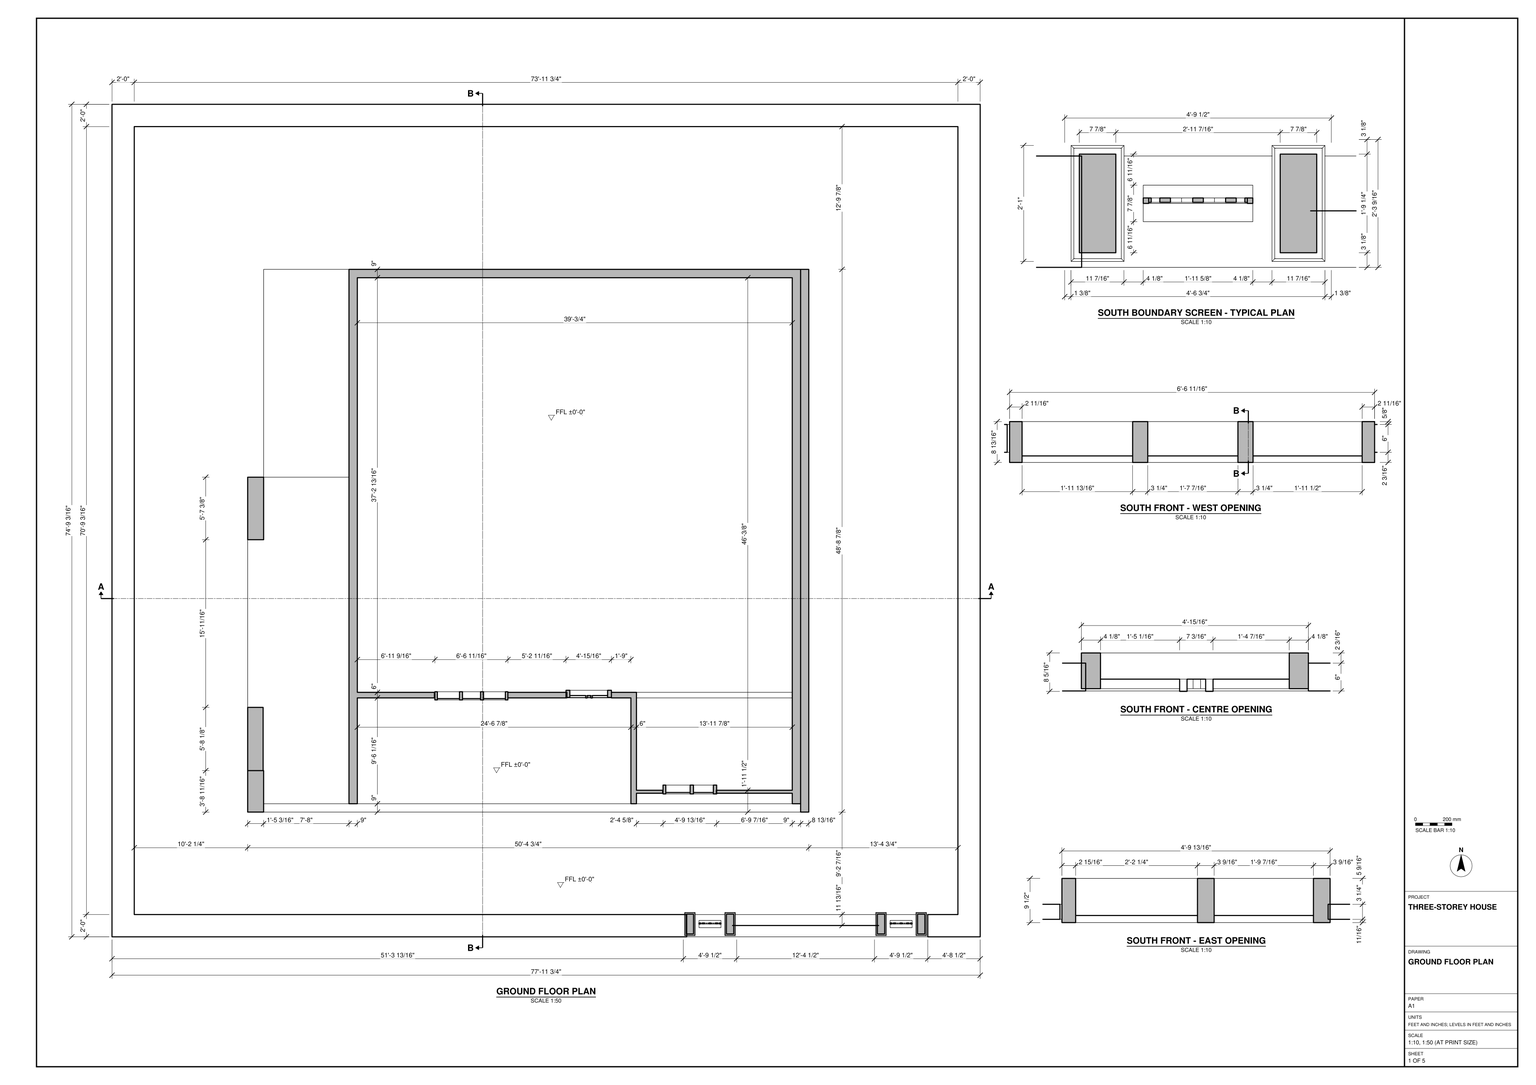
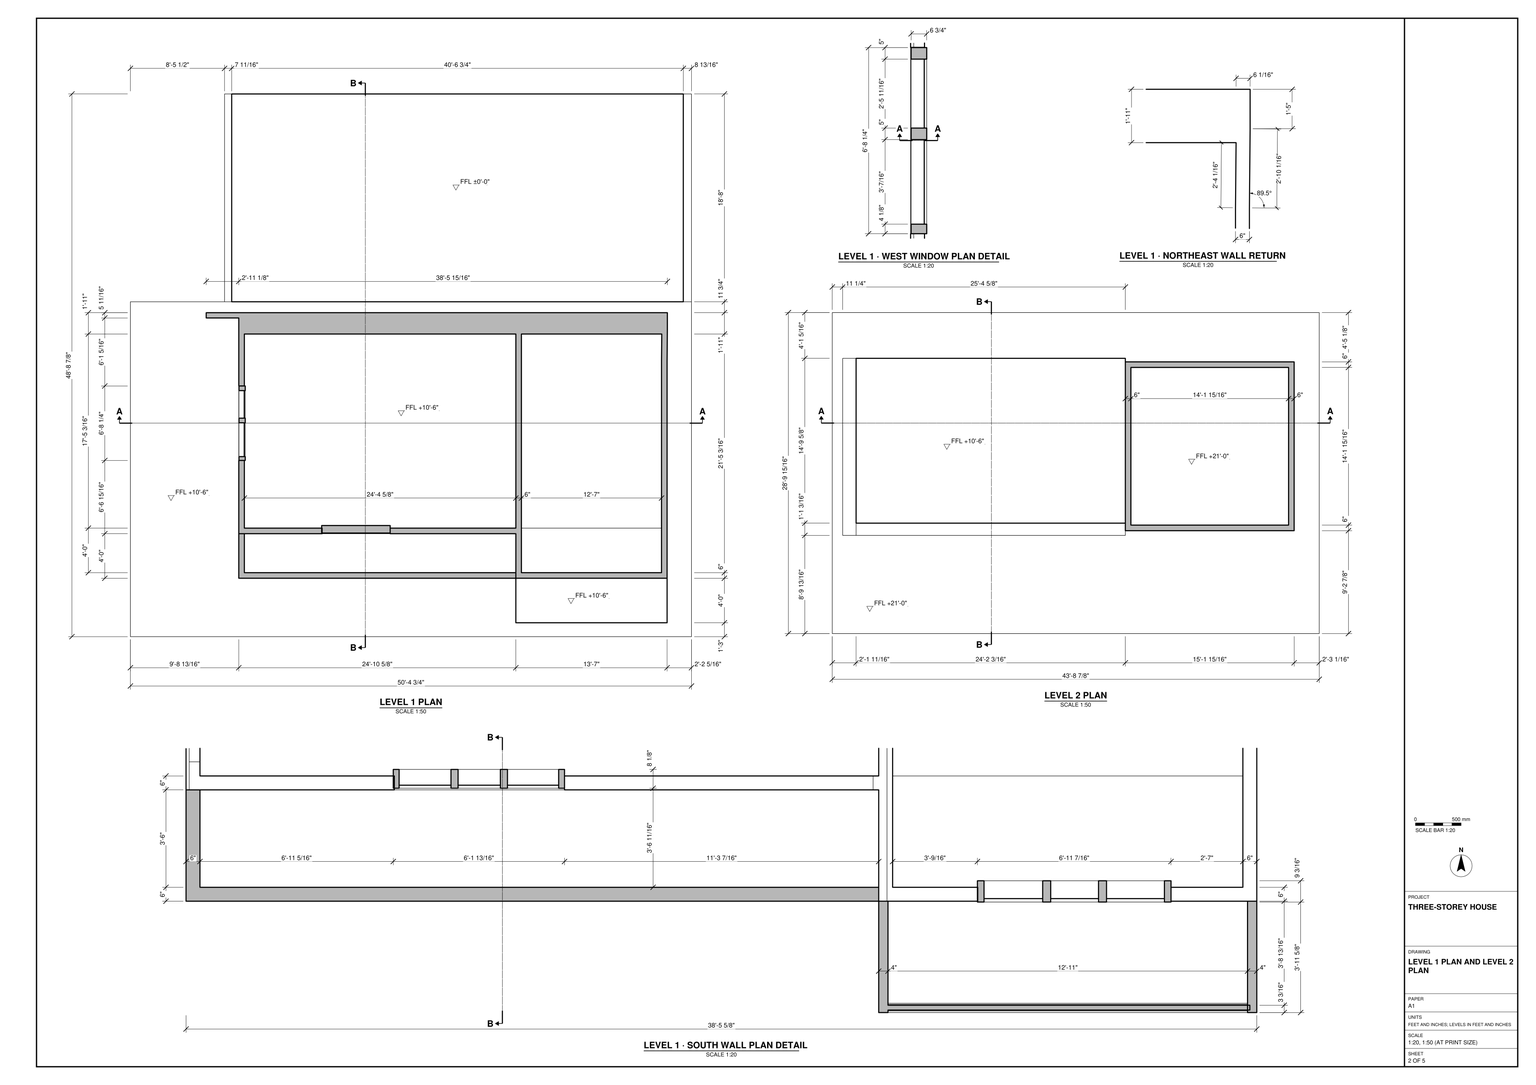
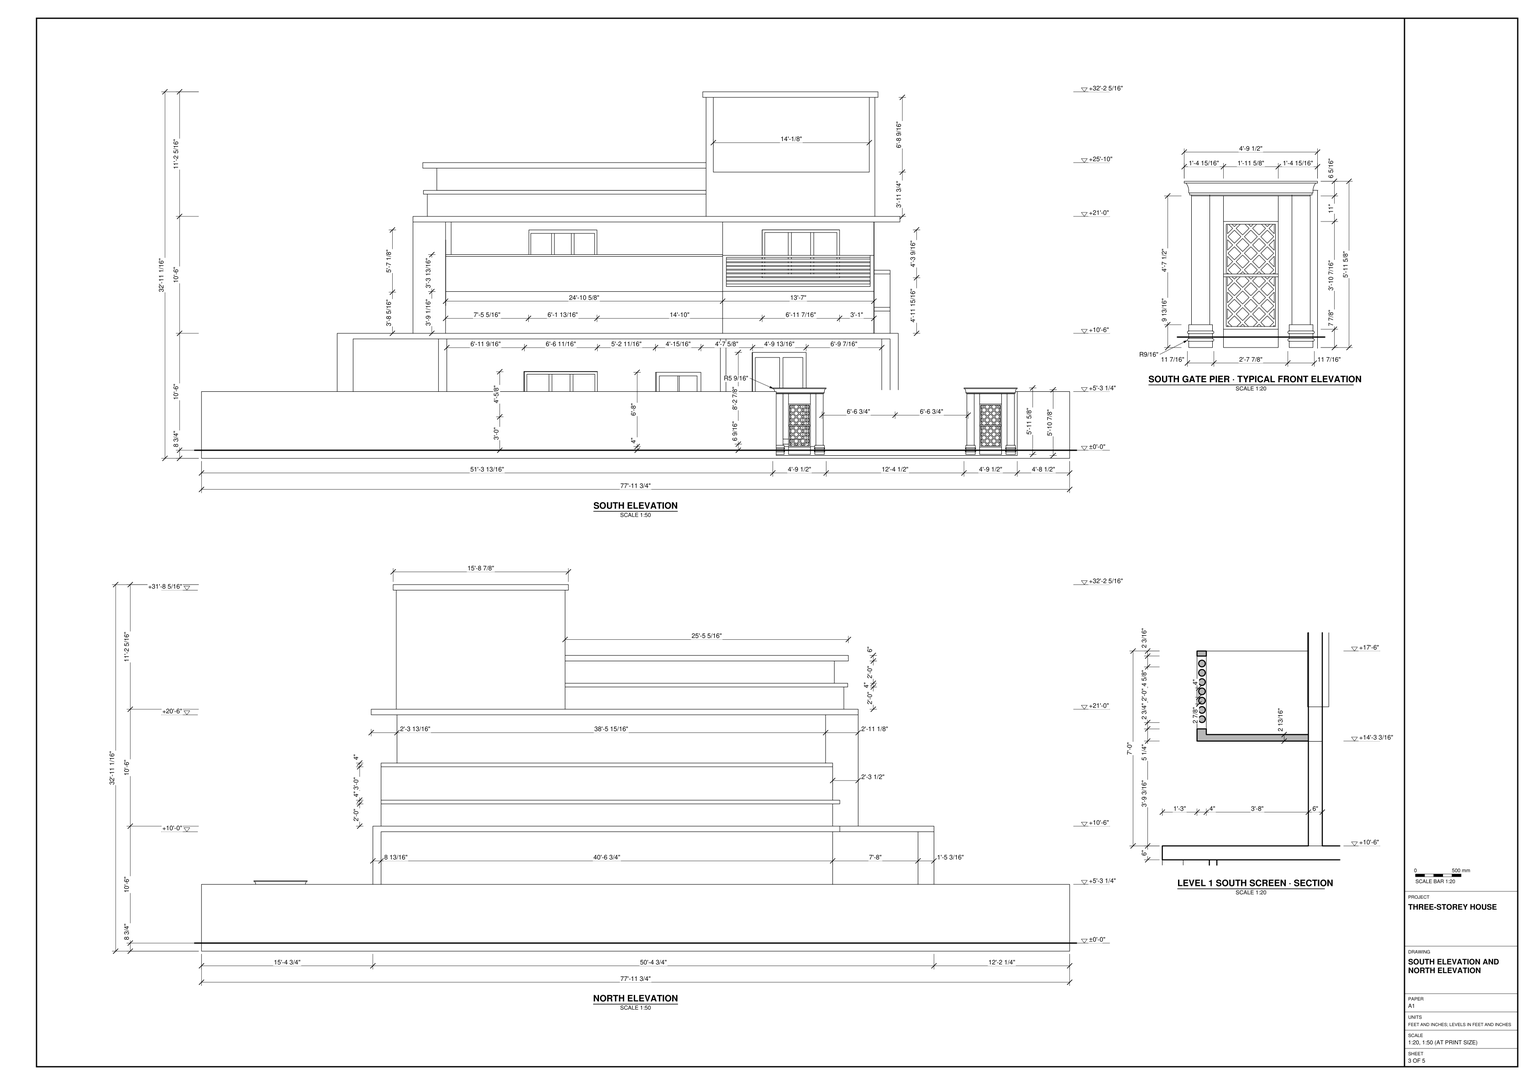
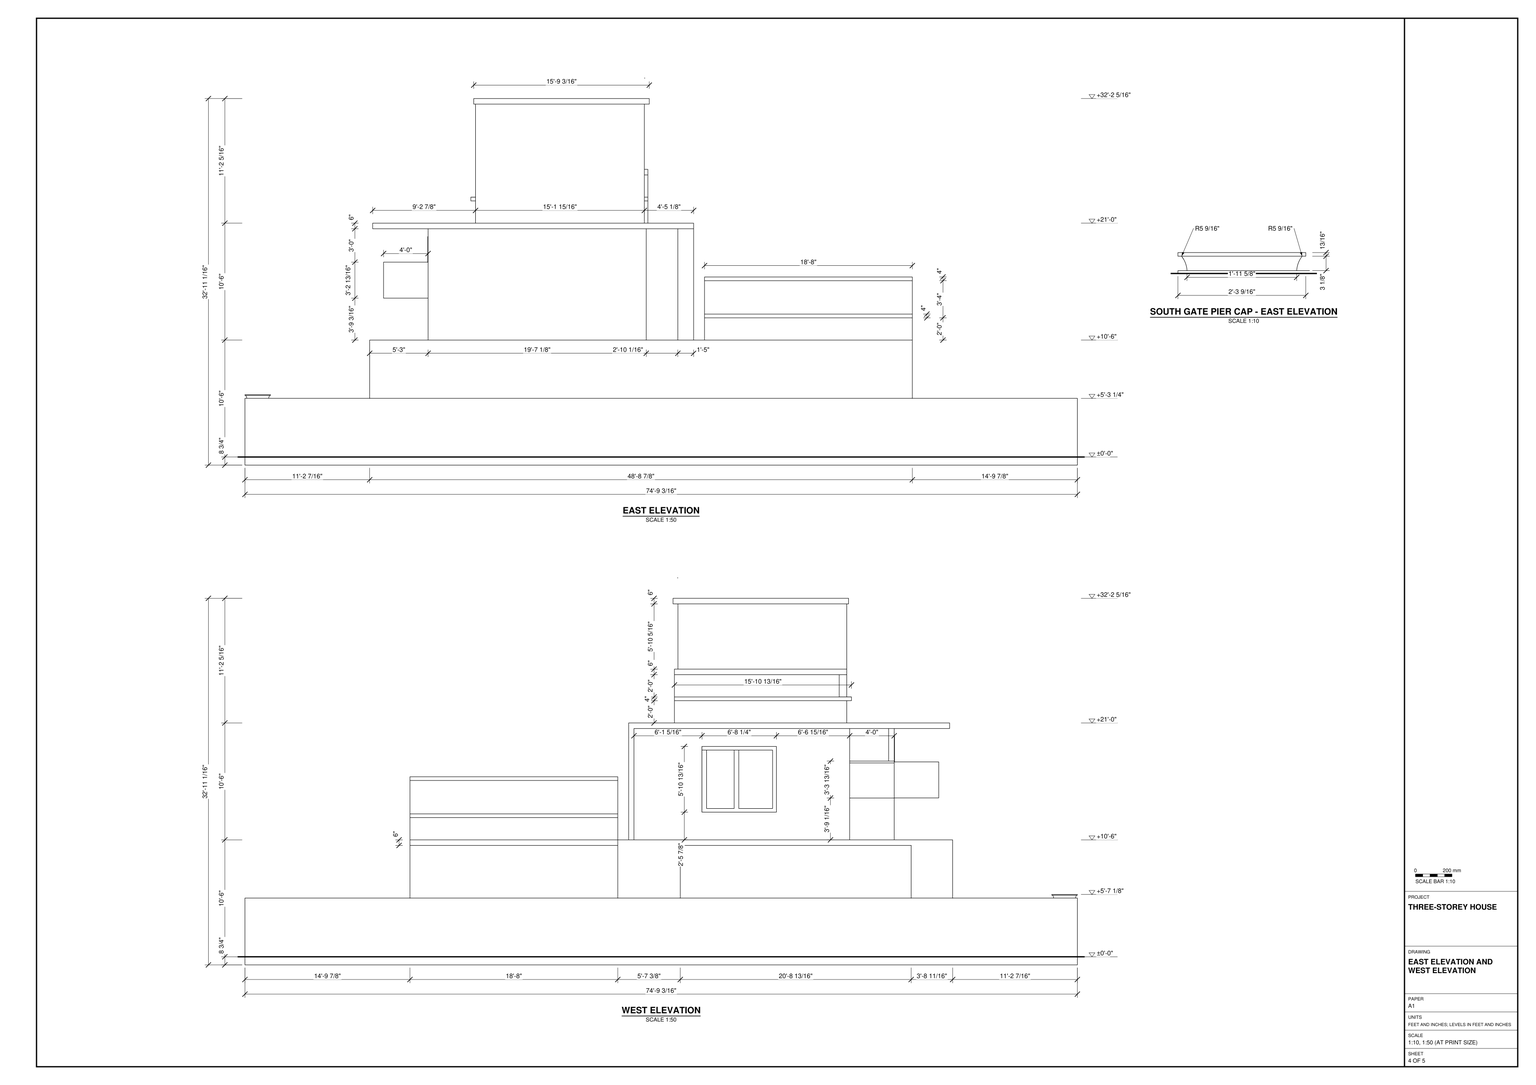
Build the house and its site in SketchUp from task_files/diagram_01.pdf. Work in feet and inches. The full model, including the site boundary, measures 77'-11 3/4" east to west, 74'-9 3/16" north to south and 32'-11 1/16" in height. Set the finished floor levels to ±0'-0", +10'-6" and +21'-0".

Use the ground floor plan to position the house within the boundary walls. Model the stepped south frontage, its framed openings and the slab projection with supports on the west side. Along the south boundary, place the two lattice screens between their capped piers as shown in the plan and elevation. Follow the drawn wall thicknesses, including the 9" ground floor exterior walls and the 6" walls where indicated, rather than using one thickness throughout.

Use the upper floor plans to locate the slabs, wall returns and setbacks. On the first upper floor, distinguish the solid balcony front from the projecting section with horizontal screening. On the top floor, place the taller enclosure to the east of the lower roof and carry the projecting flat roof edges around the volumes as drawn.

Keep walls, slabs, roofs and any furniture or joinery pieces in separate groups or components, and use components for repeated parts. Any decor or loose items shown may be represented by suitable library components. Save one SketchUp model as output_files/three_storey_house_and_its_walled_site.skp.

# SketchUp Ruby script. Lengths in inches.
U = 1.inch
M = Sketchup.active_model
def pt(a) = Geom::Point3d.new(a.map { |v| v * U })
def face(e, loops, mat)
  f = e.add_face(loops[0].map { |a| pt(a) })
  loops[1..].each { |l| e.add_face(l.map { |a| pt(a) }).erase! }
  f.material = f.back_material = mat if mat
  f
end
# faces: each face lists its corners as indices into pts; further lists are holes
def faces(e, pts, list, mat = nil) = list.each { |f| face(e, (f[0].is_a?(Array) ? f : [f]).map { |l| l.map { |i| pts[i] } }, mat) }
# xy, xz, yz: faces in a plane at the given z, y or x. An outline is a flat list of corners, or four numbers for a rectangle; further outlines are holes
def ring(l) = l.size == 4 ? [[l[0], l[1]], [l[2], l[1]], [l[2], l[3]], [l[0], l[3]]] : l.each_slice(2).to_a
def flat(e, list, mat, &to3) = list.each { |f| face(e, (f[0].is_a?(Array) ? f : [f]).map { |l| ring(l).map { |u, v| to3.(u, v) } }, mat) }
def xy(e, z, list, mat = nil) = flat(e, list, mat) { |x, y| [x, y, z] }
def xz(e, y, list, mat = nil) = flat(e, list, mat) { |x, z| [x, y, z] }
def yz(e, x, list, mat = nil) = flat(e, list, mat) { |y, z| [x, y, z] }
def lines(e, pts, list) = list.each { |a, b| e.add_line(pt(pts[a]), pt(pts[b])) }
# prism: a flat outline (further loops are holes) pulled along v
def prism(e, loops, v, mat = nil)
  f = face(e, loops, mat); d = Geom::Vector3d.new(v.map { |x| x * U })
  f.pushpull(f.normal.samedirection?(d) ? d.length : -d.length)
end
def box(e, o, s, mat = nil) = prism(e, [[o, [o[0] + s[0], o[1], o[2]], [o[0] + s[0], o[1] + s[1], o[2]], [o[0], o[1] + s[1], o[2]]]], [0, 0, s[2]], mat)
def at(x, y, z, deg = 0) = Geom::Transformation.translation(pt([x, y, z])) * Geom::Transformation.rotation(ORIGIN, Z_AXIS, deg.degrees)
def axes(o, x, y, z) = Geom::Transformation.new([*x, 0, *y, 0, *z, 0, *pt(o).to_a, 1])
def part(name) = M.definitions.add(name)
# library, detail: a bought-in or finely detailed component or shape, given as its bounding box
def library(name, o, s) = part(name).tap { |d| box(d.entities, o, s) }
def detail(e, o, s) = box(e.add_group.entities, o, s)
def put(e, d, t, mat = nil) = e.add_instance(d, t).tap { |i| i.material = mat if mat }
def group(e, t, mat = nil) = e.add_group.tap { |g| g.transformation = t; g.material = mat if mat }.entities
root = M.entities
M.materials.add("[Beadboard]").color = [218, 143, 90]
M.materials.add("[Color A07]").color = [129, 129, 129]
M.materials.add("[Color C08]").color = [102, 51, 0]
M.materials.add("[Color D01]").color = [255, 242, 204]
M.materials.add("[Color D05]").color = [255, 191, 0]
M.materials.add("[Color D06]").color = [204, 153, 0]
M.materials.add("[Color E01]").color = [255, 255, 204]
M.materials.add("[Color F07]").color = [76, 153, 0]
M.materials.add("[Color M03]").color = [170, 170, 170]
M.materials.add("[Color M04]").color = [142, 142, 142]
M.materials.add("[Color M06]").color = [86, 86, 86]
M.materials.add("[Marble Carrara Gold Floor Tile]").color = [225, 223, 217]
M.materials.add("[Stone Sandstone Ashlar Light]").color = [206, 178, 128]
M.materials.add("[Tile Navy]1").color = [43, 47, 58]
M.materials.add("[Translucent Glass Blue]").color = [100, 149, 237]
M.materials["[Translucent Glass Blue]"].alpha = 0.5
M.materials.add("[Wood Bamboo]").color = [177, 105, 43]
M.materials.add("[Wood Floor Parquet]").color = [145, 89, 39]
c1 = library("Group\#1",[0,0,0],[48,8.8125,84])
c2 = library("Group\#2",[0,0,0],[59.16,6.625,36.5625])
c3 = library("Group\#4",[0,0,0],[59.16,6.625,36.5625])
c4 = part("Group\#3")
xy(c4.entities,0,[[0,0,52.48,8.8125]])
xy(c4.entities,2.6875,[[2.6875,0,26.52,1.41],[29.78,0,49.22,1.41],[2.6875,1.41,26.52,8.8125],[29.78,1.41,49.22,8.8125]],"[Color C08]")
xy(c4.entities,45.9375,[[2.6875,0,26.52,1.41],[29.78,0,49.22,1.41],[2.6875,1.41,26.52,8.8125],[29.78,1.41,49.22,8.8125]],"[Color C08]")
xy(c4.entities,48.63,[[0,0,52.48,8.8125]])
xz(c4.entities,0,[[[0,0,52.48,48.63],[2.6875,2.6875,2.6875,45.9375,26.52,45.9375,26.52,2.6875,29.78,2.6875,29.78,45.9375,49.22,45.9375,49.22,2.6875]]],"[Color C08]")
xz(c4.entities,1.41,[[2.6875,2.6875,26.52,45.9375],[29.78,2.6875,49.22,45.9375]],"[Translucent Glass Blue]")
xz(c4.entities,8.8125,[[[0,0,0,48.63,52.48,48.63,52.48,45.9375,29.78,45.9375,29.78,2.6875,49.22,2.6875,49.22,45.9375,52.48,45.9375,52.48,0],[2.6875,2.6875,26.52,45.9375]]],"[Color C08]")
yz(c4.entities,0,[[0,0,8.8125,48.63]])
yz(c4.entities,2.6875,[[0,2.6875,1.41,45.9375],[1.41,2.6875,8.8125,45.9375]],"[Color C08]")
yz(c4.entities,26.52,[[0,2.6875,1.41,45.9375],[1.41,2.6875,8.8125,45.9375]],"[Color C08]")
yz(c4.entities,29.78,[[0,2.6875,1.41,45.9375],[1.41,2.6875,8.8125,45.9375]],"[Color C08]")
yz(c4.entities,49.22,[[0,2.6875,1.41,45.9375],[1.41,2.6875,8.8125,45.9375]],"[Color C08]")
yz(c4.entities,52.48,[[0,0,8.8125,48.63]],"[Color C08]")
p = [[29.78,8.8125,45.9375],[26.52,8.8125,45.9375]]
lines(c4.entities,p,[[0,1]])
c5 = part("Group\#5")
yz(c5.entities,0,[[0,-1.18,78.74,69.69]],"[Color A07]")
c6 = library("ة\#3",[1.38,1.28,0],[11.42,25,68.9])
c7 = library("ة\#2",[-43.31,0,0],[57.48,27.56,71.65])
c8 = part("Group\#58")
box(c8.entities,[0,5.91,0],[7.875,23.62,7.875])
c9 = part("Group\#56")
box(c9.entities,[0,5.91,0],[7.875,23.62,11.02])
c10 = library("Group\#57",[0,0,0],[23.62,1.18,46.46])
xy(root,-8.75,[[[0,0,935.75,897.1875],[24,24,911.75,873.1875]],[24,24,911.75,873.1875]])
xy(root,-5.6875,[[619.4375,0,879.27,24]],"[Stone Sandstone Ashlar Light]")
xy(root,0,[[146.25,134.4375,163.4375,179.14],[[163.4375,134.4375,742.1875,134.4375,742.1875,719.3125,163.4375,719.3125,163.4375,427.97,146.25,427.97,146.25,179.14,163.4375,179.14],[264.4375,263.5,733.1875,710.3125],[264.4375,143.4375,559.29,257.5],[565.29,143.4375,733.1875,257.5]],[742.1875,134.4375,751,719.3125],[565.29,157.96,733.1875,257.5],[264.4375,263.5,733.1875,710.3125],
  [146.25,427.97,163.4375,495.34]])
xy(root,0,[[264.4375,143.4375,559.29,257.5]],"[Color D01]")
xy(root,0,[[[24,24,911.75,873.1875],[146.25,134.4375,146.25,495.34,163.4375,495.34,163.4375,719.3125,751,719.3125,751,134.4375]]],"[Color F07]")
xy(root,0,[[565.29,143.4375,733.1875,154.72]],"[Color M03]")
xy(root,4,[[255.4375,143.4375,255.4375,719.3125,742.1875,719.3125,742.1875,143.4375,733.1875,143.4375,733.1875,710.3125,264.4375,710.3125,264.4375,263.5,490.29,263.5,490.29,257.5,264.4375,257.5,264.4375,143.4375],[559.29,143.4375,559.29,257.5,538.29,257.5,538.29,263.5,565.29,263.5,565.29,143.4375],[490.29,257.5,538.29,263.5],[565.29,257.5,733.1875,263.5]])
xy(root,4,[[163.4375,143.4375,255.4375,143.4375,255.4375,495.34,163.4375,495.34,163.4375,427.97,146.25,427.97,146.25,247.29,162.89,247.29,162.89,179.14,163.4375,179.14],[163.4375,495.34,255.4375,719.3125]],"[Color D01]")
xy(root,4,[[163.4375,134.4375,742.1875,143.4375]],"[Color M03]")
xy(root,6.56,[[593.49,154.72,651.31,157.96]])
xy(root,36,[[347.48,257.5,426.68,263.5]])
xy(root,52,[[146.25,179.14,162.89,247.29]],"[Color D01]")
xy(root,63.25,[[0,0,619.4375,0,619.4375,24,24,24,24,873.1875,911.75,873.1875,911.75,24,879.27,24,879.27,0,935.75,0,935.75,897.1875,0,897.1875]],"[Stone Sandstone Ashlar Light]")
xy(root,84,[[490.29,257.5,538.29,263.5]])
xy(root,84.95,[[347.48,257.5,426.68,263.5]])
xy(root,105.44,[[593.49,154.72,651.31,157.96]])
xy(root,120,[[163.4375,134.4375,163.4375,179.14,146.25,179.14,146.25,427.97,163.4375,427.97,163.4375,495.34,255.4375,495.34,255.4375,134.4375],[255.4375,134.4375,264.4375,143.4375],[264.4375,134.4375,559.29,257.5],[559.29,134.4375,565.29,143.4375],[565.29,134.4375,733.1875,154.72],
  [733.1875,134.4375,742.1875,143.4375],[255.4375,143.4375,264.4375,143.4375,264.4375,710.3125,733.1875,710.3125,733.1875,143.4375,742.1875,143.4375,742.1875,719.3125,255.4375,719.3125],[559.29,143.4375,559.29,257.5,264.4375,257.5,264.4375,263.5,565.29,263.5,565.29,157.96,733.1875,157.96,733.1875,154.72,565.29,154.72,565.29,143.4375],[565.29,157.96,565.29,263.5,264.4375,263.5,264.4375,710.3125,733.1875,710.3125,733.1875,157.96],[247.75,495.34,255.4375,719.3125]])
xy(root,126,[[269.09,203.41,561.71,245.41],[567.71,203.41,718.71,251.41],[269.09,251.41,561.71,460.6],[567.71,251.41,718.71,251.41,718.71,432.53,718.96,460.6,567.71,460.6],[255.4375,495.34,742.1875,719.3125]])
xy(root,126,[[[146.25,134.4375,751,495.34],[263.09,197.41,263.09,477.91,227.96,477.91,227.96,483.6,725.02,483.6,725.02,466.6,724.71,432.51,724.71,197.41]],[247.75,495.34,255.4375,719.3125],[742.1875,495.34,751,719.3125]],"[Color M04]")
xy(root,150,[[247.75,495.34,255.4375,719.3125],[255.4375,495.34,742.1875,719.3125]])
xy(root,154,[[255.4375,495.34,742.1875,719.3125]])
xy(root,154,[[247.75,495.34,255.4375,719.3125]],"[Color M04]")
xy(root,155.86,[[263.09,324.36,269.09,404.68]])
xy(root,170.23,[[352.88,245.41,426.25,251.41]],"[Color D01]")
xy(root,171.0625,[[263.09,197.41,263.09,245.41,269.09,245.41,269.09,203.41,561.71,203.41,561.71,197.41]])
xy(root,171.1875,[[561.71,149.41,724.71,197.41]])
xy(root,174,[[565.71,153.41,720.71,197.41]],"[Color M04]")
xy(root,176.44,[[565.71,149.41,720.71,153.41]],"[Color M03]")
xy(root,185.96,[[604.4,197.41,687.73,203.41]])
xy(root,190,[[255.4375,495.34,742.1875,719.3125]])
xy(root,194,[[255.4375,495.34,742.1875,719.3125]],"[Color M04]")
xy(root,207.83,[[565.71,149.41,720.71,153.41]])
xy(root,208.875,[[263.09,197.41,263.09,245.41,269.09,245.41,269.09,203.41,561.71,203.41,561.71,197.41]],"[Wood Bamboo]")
xy(root,210,[[561.71,149.41,720.71,149.41,720.71,153.41,565.71,153.41,565.71,197.41,561.71,197.41],[720.71,149.41,724.71,197.41]],"[Color M04]")
xy(root,210.875,[[263.09,197.41,561.71,197.41,561.71,203.41,269.09,203.41,269.09,245.41,263.09,245.41]],"[Wood Bamboo]")
xy(root,226.68,[[263.09,324.36,269.09,404.68]])
xy(root,237.42,[[352.88,245.41,426.25,251.41]],"[Color D01]")
xy(root,237.46,[[604.4,197.41,687.73,203.41]])
xy(root,246,[[227.96,137.66,227.96,245.41,561.71,245.41,561.71,197.41,724.71,197.41,724.71,432.51,725.02,466.6,725.02,483.6,752.83,483.6,752.83,137.66],[[561.71,197.41,561.71,245.41,263.09,245.41,263.09,251.41,561.71,251.41,561.71,460.6,263.09,460.6,263.09,483.6,725.02,483.6,725.02,466.6,724.71,432.51,724.71,197.41],[567.71,203.41,718.71,251.41]],[567.71,203.41,718.71,251.41],[227.96,245.41,263.09,251.41],[227.96,251.41,263.09,460.6],
  [263.09,251.41,269.09,460.6],[269.09,251.41,561.71,460.6],[227.96,460.6,263.09,477.91]])
xy(root,252,[[243.41,248.54,543.85,434.29],[[543.85,248.54,725.79,430.48],[549.85,254.54,719.79,424.48]],[549.85,254.54,719.79,424.48]])
xy(root,252,[[[227.96,137.66,752.83,483.6],[243.41,248.54,243.41,434.29,543.85,434.29,543.85,430.48,725.79,430.48,725.79,248.54]]],"[Color M03]")
xy(root,276,[[239.22,243.48,243.41,434.29],[243.41,243.48,543.85,248.54],[243.41,248.54,543.85,434.29]])
xy(root,280,[[253.66,256.67,543.85,434.29]])
xy(root,280,[[239.22,243.48,253.66,434.29]],"[Color M03]")
xy(root,280.0625,[[253.66,243.48,543.85,256.67]],"[Color M03]")
xy(root,304,[[238.53,248.54,253.66,434.29],[253.66,248.54,543.85,256.67],[253.66,256.67,543.85,434.29]])
xy(root,310,[[238.53,248.54,543.85,434.29]],"[Color M03]")
xy(root,380.3125,[[540.29,246.61,729.16,248.54],[540.29,248.54,543.85,254.54],[543.85,248.54,725.79,254.54],[725.79,248.54,729.16,254.54],[540.29,254.54,543.85,435.79],
  [543.85,254.54,549.85,430.48],[719.79,254.54,725.79,430.48],[725.79,254.54,729.16,435.79],[549.85,424.48,719.79,430.48],[543.85,430.48,549.85,435.79],
  [549.85,430.48,719.79,435.79],[719.79,430.48,725.79,435.79]])
xy(root,386.3125,[[540.29,246.61,729.16,435.79]],"[Beadboard]")
xz(root,0,[[0,-8.75,935.75,-8.75,935.75,63.25,879.27,63.25,879.27,-5.6875,619.4375,-5.6875,619.4375,63.25,0,63.25]],"[Stone Sandstone Ashlar Light]")
xz(root,24,[[619.4375,-5.6875,879.27,0],[879.27,0,911.75,63.25]])
xz(root,24,[[24,-8.75,24,0,619.4375,0,619.4375,-5.6875,879.27,-5.6875,879.27,0,911.75,0,911.75,-8.75]],"[Color D01]")
xz(root,24,[[24,0,619.4375,63.25]],"[Stone Sandstone Ashlar Light]")
xz(root,134.4375,[[146.25,0,163.4375,0,163.4375,120,742.1875,120,742.1875,0,751,0,751,126,146.25,126],[163.4375,0,742.1875,4]],"[Color M03]")
xz(root,137.66,[[227.96,246,752.83,252]],"[Color M03]")
xz(root,143.4375,[[264.4375,0,559.29,4],[559.29,0,559.29,4,565.29,4],[565.29,0,733.1875,4]])
xz(root,143.4375,[[733.1875,4,742.1875,120]],"[Color D06]")
xz(root,143.4375,[[255.4375,4,264.4375,120],[559.29,4,565.29,120]],"[Color M04]")
xz(root,149.41,[[561.71,171.1875,724.71,171.1875,724.71,210,720.71,210,720.71,176.44,565.71,176.44,565.71,207.83,720.71,207.83,720.71,210,561.71,210]],"[Color M03]")
xz(root,153.41,[[565.71,174,720.71,176.44],[565.71,207.83,720.71,210]])
xz(root,154.72,[[[565.29,0,733.1875,120],[593.49,6.56,651.31,105.44]]],"[Color D06]")
xz(root,157.96,[[[565.29,0,733.1875,120],[593.49,6.56,651.31,105.44]]])
xz(root,179.14,[[146.25,0,146.25,52,162.89,52,162.89,4,163.4375,4,163.4375,0]])
xz(root,179.14,[[162.89,4,162.89,52,146.25,52,146.25,120,163.4375,120,163.4375,4]],"[Color M04]")
xz(root,197.41,[[561.71,171.1875,561.71,210,565.71,210,565.71,174,720.71,174,720.71,210,724.71,210,724.71,171.1875]])
xz(root,197.41,[[263.09,126,561.71,171.0625],[561.71,126,724.71,171.1875]],"[Color D01]")
xz(root,197.41,[[[565.71,174,720.71,174,720.71,210,724.71,210,724.71,246,561.71,246,561.71,210,565.71,210],[604.4,185.96,687.73,237.46]]],"[Color D06]")
xz(root,197.41,[[263.09,171.0625,561.71,208.875]],"[Translucent Glass Blue]")
xz(root,197.41,[[263.09,208.875,561.71,210.875]],"[Wood Bamboo]")
xz(root,203.41,[[269.09,126,561.71,171.0625],[[567.71,126,718.71,246],[604.4,185.96,687.73,237.46]]])
xz(root,203.41,[[269.09,171.0625,561.71,208.875]],"[Translucent Glass Blue]")
xz(root,203.41,[[269.09,208.875,561.71,210.875]],"[Wood Bamboo]")
xz(root,243.48,[[239.22,276,543.85,276,543.85,280.0625,253.66,280.0625,253.66,280,239.22,280]],"[Color M03]")
xz(root,245.41,[[263.09,171.0625,269.09,208.875]])
xz(root,245.41,[[[269.09,126,561.71,246],[352.88,170.23,426.25,237.42]],[263.09,210.875,269.09,246]],"[Color D06]")
xz(root,245.41,[[263.09,208.875,269.09,210.875]],"[Wood Bamboo]")
xz(root,246.61,[[540.29,380.3125,729.16,386.3125]],"[Beadboard]")
xz(root,247.29,[[146.25,4,162.89,52]],"[Color D01]")
xz(root,248.54,[[243.41,252,543.85,276],[543.85,252,725.79,252,725.79,380.3125,719.79,380.3125,719.79,299.75,551.67,299.75,551.67,380.3125,543.85,380.3125]],"[Color D01]")
xz(root,248.54,[[238.53,304,543.85,310]],"[Color M03]")
xz(root,248.54,[[551.67,299.75,719.79,380.3125]],"[Translucent Glass Blue]")
xz(root,251.41,[[[269.09,126,561.71,246],[352.88,170.23,426.25,237.42]]])
xz(root,254.54,[[549.85,252,719.79,289.37]])
xz(root,254.54,[[549.85,289.37,719.79,380.3125]],"[Translucent Glass Blue]")
xz(root,256.67,[[253.66,280,543.85,280.0625]])
xz(root,256.67,[[253.66,280.0625,543.85,304]],"[Wood Floor Parquet]")
xz(root,257.5,[[565.29,0,733.1875,4]])
xz(root,257.5,[[[264.4375,4,490.29,4,490.29,84,538.29,84,538.29,4,559.29,4,559.29,120,264.4375,120],[347.48,36,426.68,84.95]]],"[Color D06]")
xz(root,257.5,[[264.4375,0,559.29,4]],"[Color M04]")
xz(root,263.5,[[264.4375,0,733.1875,4],[[264.4375,4,264.4375,120,565.29,120,565.29,4,538.29,4,538.29,84,490.29,84,490.29,4],[347.48,36,426.68,84.95]]])
xz(root,324.36,[[263.09,155.86,269.09,226.68]])
xz(root,404.68,[[263.09,155.86,269.09,226.68]])
xz(root,424.48,[[549.85,252,719.79,380.3125]])
xz(root,427.97,[[146.25,0,163.4375,4]])
xz(root,427.97,[[146.25,4,163.4375,120]],"[Color M04]")
xz(root,430.48,[[543.85,252,725.79,380.3125]],"[Color D01]")
xz(root,434.29,[[243.41,252,543.85,276],[253.66,280,543.85,304]],"[Color D01]")
xz(root,434.29,[[239.22,276,543.85,280],[238.53,304,543.85,310]],"[Color M03]")
xz(root,435.79,[[540.29,380.3125,729.16,386.3125]],"[Beadboard]")
xz(root,460.6,[[269.09,126,561.71,246],[567.71,126,718.96,246]])
xz(root,477.91,[[227.96,126,263.09,246]],"[Color M03]")
xz(root,483.6,[[263.09,126,725.02,246]],"[Color D01]")
xz(root,483.6,[[227.96,126,263.09,246],[227.96,246,752.83,252]],"[Color M03]")
xz(root,495.34,[[255.4375,126,742.1875,150],[255.4375,154,742.1875,190]],"[Color D01]")
xz(root,495.34,[[146.25,120,247.75,126]],"[Color M03]")
xz(root,495.34,[[146.25,0,163.4375,120],[247.75,150,742.1875,154],[255.4375,190,742.1875,194]],"[Color M04]")
xz(root,710.3125,[[264.4375,0,733.1875,4],[264.4375,4,733.1875,120]])
xz(root,719.3125,[[255.4375,126,742.1875,150],[255.4375,154,742.1875,190]],"[Color D01]")
xz(root,719.3125,[[255.4375,4,742.1875,120]],"[Color D05]")
xz(root,719.3125,[[163.4375,0,742.1875,4]],"[Color E01]")
xz(root,719.3125,[[742.1875,0,742.1875,120,247.75,120,247.75,126,751,126,751,0],[247.75,150,742.1875,154],[255.4375,190,742.1875,194]],"[Color M04]")
xz(root,873.1875,[[24,-8.75,911.75,0]],"[Color D01]")
xz(root,873.1875,[[24,0,911.75,63.25]],"[Stone Sandstone Ashlar Light]")
xz(root,897.1875,[[0,-8.75,935.75,63.25]],"[Stone Sandstone Ashlar Light]")
yz(root,0,[[0,-8.75,897.1875,63.25]],"[Stone Sandstone Ashlar Light]")
yz(root,24,[[24,-8.75,873.1875,0]],"[Color D01]")
yz(root,24,[[24,0,873.1875,63.25]],"[Stone Sandstone Ashlar Light]")
yz(root,146.25,[[179.14,0,179.14,52,247.29,52,247.29,4,427.97,4,427.97,0]],"[Color D01]")
yz(root,146.25,[[134.4375,0,134.4375,126,495.34,126,495.34,0,427.97,0,427.97,120,179.14,120,179.14,0]],"[Color M03]")
yz(root,162.89,[[179.14,4,247.29,52]],"[Color D01]")
yz(root,163.4375,[[134.4375,0,179.14,4],[427.97,0,495.34,4],[427.97,4,495.34,120]])
yz(root,163.4375,[[495.34,0,719.3125,4]],"[Color D01]")
yz(root,163.4375,[[134.4375,4,179.14,120]],"[Color M04]")
yz(root,227.96,[[477.91,126,477.91,246,137.66,246,137.66,252,483.6,252,483.6,126]],"[Color M03]")
yz(root,238.53,[[248.54,304,434.29,310]],"[Color M03]")
yz(root,239.22,[[243.48,276,434.29,280]],"[Color M03]")
yz(root,243.41,[[248.54,252,434.29,276]],"[Color D01]")
yz(root,247.75,[[495.34,120,719.3125,126],[495.34,150,719.3125,154]],"[Color M04]")
yz(root,253.66,[[243.48,280,256.67,280.0625]])
yz(root,253.66,[[256.67,280,434.29,304]],"[Wood Floor Parquet]")
yz(root,255.4375,[[495.34,126,719.3125,150],[495.34,154,719.3125,190]],"[Color D01]")
yz(root,255.4375,[[143.4375,4,719.3125,120]],"[Color D06]")
yz(root,255.4375,[[495.34,190,719.3125,194]],"[Color M04]")
yz(root,263.09,[[197.41,126,245.41,171.0625]],"[Color D01]")
yz(root,263.09,[[[245.41,126,477.91,246],[324.36,155.86,404.68,226.68]]],"[Color D06]")
yz(root,263.09,[[197.41,171.0625,245.41,208.875]],"[Translucent Glass Blue]")
yz(root,263.09,[[197.41,208.875,245.41,210.875]],"[Wood Bamboo]")
yz(root,264.4375,[[263.5,0,710.3125,4],[263.5,4,710.3125,120]])
yz(root,264.4375,[[143.4375,4,257.5,120]],"[Color D06]")
yz(root,264.4375,[[143.4375,0,257.5,4]],"[Color M04]")
yz(root,269.09,[[203.41,126,245.41,171.0625],[[251.41,126,460.6,246],[324.36,155.86,404.68,226.68]]])
yz(root,269.09,[[203.41,171.0625,245.41,208.875]],"[Translucent Glass Blue]")
yz(root,269.09,[[203.41,208.875,245.41,210.875]],"[Wood Bamboo]")
yz(root,347.48,[[257.5,36,263.5,84.95]])
yz(root,352.88,[[245.41,170.23,251.41,237.42]],"[Color D01]")
yz(root,426.25,[[245.41,170.23,251.41,237.42]],"[Color D01]")
yz(root,426.68,[[257.5,36,263.5,84.95]])
yz(root,490.29,[[257.5,4,263.5,84]])
yz(root,538.29,[[257.5,4,263.5,84]])
yz(root,540.29,[[246.61,380.3125,435.79,386.3125]],"[Beadboard]")
yz(root,543.85,[[248.54,252,430.48,276],[243.48,276,248.54,280.0625],[248.54,276,248.54,280.0625,256.67,280.0625,256.67,280,430.48,280,430.48,276],[256.67,280,430.48,304],[248.54,280.0625,256.67,304],
  [248.54,304,430.48,310]])
yz(root,543.85,[[430.48,252,434.29,276],[430.48,276,434.29,280],[430.48,280,434.29,304],[430.48,304,434.29,310],[248.54,310,430.48,380.3125]],"[Color D01]")
yz(root,549.85,[[254.54,252,424.48,380.3125]])
yz(root,559.29,[[143.4375,4,257.5,120]],"[Color D06]")
yz(root,559.29,[[143.4375,0,257.5,4]],"[Color M04]")
yz(root,561.71,[[251.41,126,460.6,246],[197.41,171.0625,203.41,208.875]])
yz(root,561.71,[[203.41,126,245.41,246],[197.41,210.875,203.41,246]],"[Color D06]")
yz(root,561.71,[[149.41,171.1875,197.41,210]],"[Color M03]")
yz(root,561.71,[[197.41,208.875,203.41,210.875]],"[Wood Bamboo]")
yz(root,565.29,[[143.4375,0,154.72,4],[154.72,0,157.96,4],[157.96,0,257.5,4],[143.4375,4,154.72,120],[157.96,4,263.5,120]])
yz(root,565.71,[[153.41,174,197.41,210],[[149.41,176.44,153.41,207.83],[151.53,183.18,151.16,183.23,150.81,183.37,150.51,183.6,150.28,183.9,150.14,184.25,150.09,184.62,150.14,184.99,150.28,185.34,150.51,185.63,150.81,185.86,151.16,186.01,151.53,186.06,151.9,186.01,152.25,185.86,152.55,185.63,152.77,185.34,152.92,184.99,152.97,184.62,152.92,184.25,152.77,183.9,152.55,183.6,152.25,183.37,151.9,183.23],[151.53,187.18,151.16,187.23,150.81,187.37,150.51,187.6,150.28,187.9,150.14,188.25,150.09,188.62,150.14,188.99,150.28,189.34,150.51,189.63,150.81,189.86,151.16,190.01,151.53,190.06,151.9,190.01,152.25,189.86,152.55,189.63,152.77,189.34,152.92,188.99,152.97,188.62,152.92,188.25,152.77,187.9,152.55,187.6,152.25,187.37,151.9,187.23],[151.53,191.18,151.16,191.23,150.81,191.37,150.51,191.6,150.28,191.9,150.14,192.25,150.09,192.62,150.14,192.99,150.28,193.34,150.51,193.63,150.81,193.86,151.16,194.01,151.53,194.06,151.9,194.01,152.25,193.86,152.55,193.63,152.77,193.34,152.92,192.99,152.97,192.62,152.92,192.25,152.77,191.9,152.55,191.6,152.25,191.37,151.9,191.23],[151.53,195.18,151.16,195.23,150.81,195.37,150.51,195.6,150.28,195.9,150.14,196.25,150.09,196.62,150.14,196.99,150.28,197.34,150.51,197.63,150.81,197.86,151.16,198.01,151.53,198.06,151.9,198.01,152.25,197.86,152.55,197.63,152.77,197.34,152.92,196.99,152.97,196.62,152.92,196.25,152.77,195.9,152.55,195.6,152.25,195.37,151.9,195.23],[151.53,199.18,151.16,199.23,150.81,199.37,150.51,199.6,150.28,199.9,150.14,200.25,150.09,200.62,150.14,200.99,150.28,201.34,150.51,201.63,150.81,201.86,151.16,202.01,151.53,202.06,151.9,202.01,152.25,201.86,152.55,201.63,152.77,201.34,152.92,200.99,152.97,200.62,152.92,200.25,152.77,199.9,152.55,199.6,152.25,199.37,151.9,199.23],[151.53,203.18,151.16,203.23,150.81,203.37,150.51,203.6,150.28,203.9,150.14,204.25,150.09,204.62,150.14,204.99,150.28,205.34,150.51,205.63,150.81,205.86,151.16,206.01,151.53,206.06,151.9,206.01,152.25,205.86,152.55,205.63,152.77,205.34,152.92,204.99,152.97,204.62,152.92,204.25,152.77,203.9,152.55,203.6,152.25,203.37,151.9,203.23],[151.53,179.18,151.16,179.23,150.81,179.37,150.51,179.6,150.28,179.9,150.14,180.25,150.09,180.62,150.14,180.99,150.28,181.34,150.51,181.63,150.81,181.86,151.16,182.01,151.53,182.06,151.9,182.01,152.25,181.86,152.55,181.63,152.77,181.34,152.92,180.99,152.97,180.62,152.92,180.25,152.77,179.9,152.55,179.6,152.25,179.37,151.9,179.23]]],"[Color M03]")
yz(root,567.71,[[203.41,126,251.41,246],[251.41,126,460.6,246]])
yz(root,593.49,[[154.72,6.56,157.96,105.44]])
yz(root,604.4,[[197.41,185.96,203.41,237.46]])
yz(root,619.4375,[[0,-5.6875,24,63.25]])
yz(root,651.31,[[154.72,6.56,157.96,105.44]])
yz(root,687.73,[[197.41,185.96,203.41,237.46]])
yz(root,718.71,[[203.41,126,251.41,246],[251.41,126,432.53,246]])
yz(root,719.79,[[254.54,252,424.48,380.3125]])
yz(root,720.59,[[151.53,179.18,151.9,179.23,152.25,179.37,152.55,179.6,152.77,179.9,152.92,180.25,152.97,180.62,152.92,180.99,152.77,181.34,152.55,181.63,152.25,181.86,151.9,182.01,151.53,182.06,151.16,182.01,150.81,181.86,150.51,181.63,150.28,181.34,150.14,180.99,150.09,180.62,150.14,180.25,150.28,179.9,150.51,179.6,150.81,179.37,151.16,179.23]])
yz(root,720.71,[[[149.41,176.44,153.41,207.83],[151.53,183.18,151.9,183.23,152.25,183.37,152.55,183.6,152.77,183.9,152.92,184.25,152.97,184.62,152.92,184.99,152.77,185.34,152.55,185.63,152.25,185.86,151.9,186.01,151.53,186.06,151.16,186.01,150.81,185.86,150.51,185.63,150.28,185.34,150.14,184.99,150.09,184.62,150.14,184.25,150.28,183.9,150.51,183.6,150.81,183.37,151.16,183.23],[151.53,191.18,151.9,191.23,152.25,191.37,152.55,191.6,152.77,191.9,152.92,192.25,152.97,192.62,152.92,192.99,152.77,193.34,152.55,193.63,152.25,193.86,151.9,194.01,151.53,194.06,151.16,194.01,150.81,193.86,150.51,193.63,150.28,193.34,150.14,192.99,150.09,192.62,150.14,192.25,150.28,191.9,150.51,191.6,150.81,191.37,151.16,191.23],[151.53,195.18,151.9,195.23,152.25,195.37,152.55,195.6,152.77,195.9,152.92,196.25,152.97,196.62,152.92,196.99,152.77,197.34,152.55,197.63,152.25,197.86,151.9,198.01,151.53,198.06,151.16,198.01,150.81,197.86,150.51,197.63,150.28,197.34,150.14,196.99,150.09,196.62,150.14,196.25,150.28,195.9,150.51,195.6,150.81,195.37,151.16,195.23]]],"[Color M03]")
yz(root,720.71,[[153.41,174,197.41,210]],"[Color M04]")
yz(root,721.21,[[151.53,187.18,151.9,187.23,152.25,187.37,152.55,187.6,152.77,187.9,152.92,188.25,152.97,188.62,152.92,188.99,152.77,189.34,152.55,189.63,152.25,189.86,151.9,190.01,151.53,190.06,151.16,190.01,150.81,189.86,150.51,189.63,150.28,189.34,150.14,188.99,150.09,188.62,150.14,188.25,150.28,187.9,150.51,187.6,150.81,187.37,151.16,187.23]])
yz(root,721.71,[[151.53,199.18,151.9,199.23,152.25,199.37,152.55,199.6,152.77,199.9,152.92,200.25,152.97,200.62,152.92,200.99,152.77,201.34,152.55,201.63,152.25,201.86,151.9,202.01,151.53,202.06,151.16,202.01,150.81,201.86,150.51,201.63,150.28,201.34,150.14,200.99,150.09,200.62,150.14,200.25,150.28,199.9,150.51,199.6,150.81,199.37,151.16,199.23]])
yz(root,722.71,[[151.53,203.18,151.9,203.23,152.25,203.37,152.55,203.6,152.77,203.9,152.92,204.25,152.97,204.62,152.92,204.99,152.77,205.34,152.55,205.63,152.25,205.86,151.9,206.01,151.53,206.06,151.16,206.01,150.81,205.86,150.51,205.63,150.28,205.34,150.14,204.99,150.09,204.62,150.14,204.25,150.28,203.9,150.51,203.6,150.81,203.37,151.16,203.23]])
yz(root,724.71,[[197.41,126,432.51,246]],"[Color D01]")
yz(root,724.71,[[149.41,171.1875,197.41,210]],"[Color M04]")
yz(root,725.02,[[466.6,126,483.6,246]],"[Color D01]")
yz(root,725.79,[[248.54,252,430.48,380.3125]],"[Color D01]")
yz(root,729.16,[[246.61,380.3125,435.79,386.3125]],"[Beadboard]")
yz(root,733.1875,[[154.72,0,157.96,4],[157.96,0,257.5,4],[263.5,0,710.3125,4],[157.96,4,710.3125,120]])
yz(root,733.1875,[[143.4375,0,154.72,4],[143.4375,4,154.72,120]],"[Color D05]")
yz(root,742.1875,[[134.4375,0,719.3125,4],[143.4375,4,719.3125,120]])
yz(root,742.1875,[[495.34,126,719.3125,150],[495.34,154,719.3125,190]],"[Color D01]")
yz(root,742.1875,[[134.4375,4,143.4375,120]],"[Color D05]")
yz(root,742.1875,[[495.34,150,719.3125,154],[495.34,190,719.3125,194]],"[Color M04]")
yz(root,751,[[134.4375,0,719.3125,126]],"[Color D05]")
yz(root,752.83,[[137.66,246,483.6,252]],"[Color M03]")
yz(root,879.27,[[0,-5.6875,24,63.25]])
yz(root,911.75,[[24,-8.75,873.1875,0]],"[Color D01]")
yz(root,911.75,[[24,0,873.1875,63.25]],"[Stone Sandstone Ashlar Light]")
yz(root,935.75,[[0,-8.75,897.1875,63.25]],"[Stone Sandstone Ashlar Light]")
p = [[718.96,460.6,126],[718.71,432.53,126],[718.71,432.53,246],[718.96,460.6,246],[724.71,432.51,126],[725.02,466.6,126],
  [725.02,466.6,246],[724.71,432.51,246],[565.71,150.81,179.37],[565.71,151.16,179.23],[720.59,151.16,179.23],[720.59,150.81,179.37],
  [565.71,151.53,179.18],[720.59,151.53,179.18],[565.71,151.9,179.23],[720.59,151.9,179.23],[565.71,152.25,179.37],[720.59,152.25,179.37],
  [565.71,150.51,179.6],[720.59,150.51,179.6],[565.71,152.55,179.6],[720.59,152.55,179.6],[565.71,150.28,179.9],[720.59,150.28,179.9],
  [565.71,152.77,179.9],[720.59,152.77,179.9],[565.71,150.14,180.25],[720.59,150.14,180.25],[565.71,152.92,180.25],[720.59,152.92,180.25],
  [565.71,150.09,180.62],[720.59,150.09,180.62],[565.71,152.97,180.62],[720.59,152.97,180.62],[565.71,150.14,180.99],[720.59,150.14,180.99],
  [565.71,152.92,180.99],[720.59,152.92,180.99],[565.71,150.28,181.34],[720.59,150.28,181.34],[565.71,152.77,181.34],[720.59,152.77,181.34],
  [565.71,150.51,181.63],[720.59,150.51,181.63],[565.71,152.55,181.63],[720.59,152.55,181.63],[565.71,150.81,181.86],[720.59,150.81,181.86],
  [565.71,152.25,181.86],[720.59,152.25,181.86],[565.71,151.16,182.01],[720.59,151.16,182.01],[565.71,151.9,182.01],[720.59,151.9,182.01],
  [565.71,151.53,182.06],[720.59,151.53,182.06],[565.71,150.81,183.37],[565.71,151.16,183.23],[720.71,151.16,183.23],[720.71,150.81,183.37],
  [565.71,151.53,183.18],[720.71,151.53,183.18],[565.71,151.9,183.23],[720.71,151.9,183.23],[565.71,152.25,183.37],[720.71,152.25,183.37],
  [565.71,150.51,183.6],[720.71,150.51,183.6],[565.71,152.55,183.6],[720.71,152.55,183.6],[565.71,150.28,183.9],[720.71,150.28,183.9],
  [565.71,152.77,183.9],[720.71,152.77,183.9],[565.71,150.14,184.25],[720.71,150.14,184.25],[565.71,152.92,184.25],[720.71,152.92,184.25],
  [565.71,150.09,184.62],[720.71,150.09,184.62],[565.71,152.97,184.62],[720.71,152.97,184.62],[565.71,150.14,184.99],[720.71,150.14,184.99],
  [565.71,152.92,184.99],[720.71,152.92,184.99],[565.71,150.28,185.34],[720.71,150.28,185.34],[565.71,152.77,185.34],[720.71,152.77,185.34],
  [565.71,150.51,185.63],[720.71,150.51,185.63],[565.71,152.55,185.63],[720.71,152.55,185.63],[565.71,150.81,185.86],[720.71,150.81,185.86],
  [565.71,152.25,185.86],[720.71,152.25,185.86],[565.71,151.16,186.01],[720.71,151.16,186.01],[565.71,151.9,186.01],[720.71,151.9,186.01],
  [565.71,151.53,186.06],[720.71,151.53,186.06],[565.71,150.81,187.37],[565.71,151.16,187.23],[721.21,151.16,187.23],[721.21,150.81,187.37],
  [565.71,151.53,187.18],[721.21,151.53,187.18],[565.71,151.9,187.23],[721.21,151.9,187.23],[565.71,152.25,187.37],[721.21,152.25,187.37],
  [565.71,150.51,187.6],[721.21,150.51,187.6],[565.71,152.55,187.6],[721.21,152.55,187.6],[565.71,150.28,187.9],[721.21,150.28,187.9],
  [565.71,152.77,187.9],[721.21,152.77,187.9],[565.71,150.14,188.25],[721.21,150.14,188.25],[565.71,152.92,188.25],[721.21,152.92,188.25],
  [565.71,150.09,188.62],[721.21,150.09,188.62],[565.71,152.97,188.62],[721.21,152.97,188.62],[565.71,150.14,188.99],[721.21,150.14,188.99],
  [565.71,152.92,188.99],[721.21,152.92,188.99],[565.71,150.28,189.34],[721.21,150.28,189.34],[565.71,152.77,189.34],[721.21,152.77,189.34],
  [565.71,150.51,189.63],[721.21,150.51,189.63],[565.71,152.55,189.63],[721.21,152.55,189.63],[565.71,150.81,189.86],[721.21,150.81,189.86],
  [565.71,152.25,189.86],[721.21,152.25,189.86],[565.71,151.16,190.01],[721.21,151.16,190.01],[565.71,151.9,190.01],[721.21,151.9,190.01],
  [565.71,151.53,190.06],[721.21,151.53,190.06],[565.71,150.81,191.37],[565.71,151.16,191.23],[720.71,151.16,191.23],[720.71,150.81,191.37],
  [565.71,151.53,191.18],[720.71,151.53,191.18],[565.71,151.9,191.23],[720.71,151.9,191.23],[565.71,152.25,191.37],[720.71,152.25,191.37],
  [565.71,150.51,191.6],[720.71,150.51,191.6],[565.71,152.55,191.6],[720.71,152.55,191.6],[565.71,150.28,191.9],[720.71,150.28,191.9],
  [565.71,152.77,191.9],[720.71,152.77,191.9],[565.71,150.14,192.25],[720.71,150.14,192.25],[565.71,152.92,192.25],[720.71,152.92,192.25],
  [565.71,150.09,192.62],[720.71,150.09,192.62],[565.71,152.97,192.62],[720.71,152.97,192.62],[565.71,150.14,192.99],[720.71,150.14,192.99],
  [565.71,152.92,192.99],[720.71,152.92,192.99],[565.71,150.28,193.34],[720.71,150.28,193.34],[565.71,152.77,193.34],[720.71,152.77,193.34],
  [565.71,150.51,193.63],[720.71,150.51,193.63],[565.71,152.55,193.63],[720.71,152.55,193.63],[565.71,150.81,193.86],[720.71,150.81,193.86],
  [565.71,152.25,193.86],[720.71,152.25,193.86],[565.71,151.16,194.01],[720.71,151.16,194.01],[565.71,151.9,194.01],[720.71,151.9,194.01],
  [565.71,151.53,194.06],[720.71,151.53,194.06],[565.71,150.81,195.37],[565.71,151.16,195.23],[720.71,151.16,195.23],[720.71,150.81,195.37],
  [565.71,151.53,195.18],[720.71,151.53,195.18],[565.71,151.9,195.23],[720.71,151.9,195.23],[565.71,152.25,195.37],[720.71,152.25,195.37],
  [565.71,150.51,195.6],[720.71,150.51,195.6],[565.71,152.55,195.6],[720.71,152.55,195.6],[565.71,150.28,195.9],[720.71,150.28,195.9],
  [565.71,152.77,195.9],[720.71,152.77,195.9],[565.71,150.14,196.25],[720.71,150.14,196.25],[565.71,152.92,196.25],[720.71,152.92,196.25],
  [565.71,150.09,196.62],[720.71,150.09,196.62],[565.71,152.97,196.62],[720.71,152.97,196.62],[565.71,150.14,196.99],[720.71,150.14,196.99],
  [565.71,152.92,196.99],[720.71,152.92,196.99],[565.71,150.28,197.34],[720.71,150.28,197.34],[565.71,152.77,197.34],[720.71,152.77,197.34],
  [565.71,150.51,197.63],[720.71,150.51,197.63],[565.71,152.55,197.63],[720.71,152.55,197.63],[565.71,150.81,197.86],[720.71,150.81,197.86],
  [565.71,152.25,197.86],[720.71,152.25,197.86],[565.71,151.16,198.01],[720.71,151.16,198.01],[565.71,151.9,198.01],[720.71,151.9,198.01],
  [565.71,151.53,198.06],[720.71,151.53,198.06],[565.71,150.81,199.37],[565.71,151.16,199.23],[721.71,151.16,199.23],[721.71,150.81,199.37],
  [565.71,151.53,199.18],[721.71,151.53,199.18],[565.71,151.9,199.23],[721.71,151.9,199.23],[565.71,152.25,199.37],[721.71,152.25,199.37],
  [565.71,150.51,199.6],[721.71,150.51,199.6],[565.71,152.55,199.6],[721.71,152.55,199.6],[565.71,150.28,199.9],[721.71,150.28,199.9],
  [565.71,152.77,199.9],[721.71,152.77,199.9],[565.71,150.14,200.25],[721.71,150.14,200.25],[565.71,152.92,200.25],[721.71,152.92,200.25],
  [565.71,150.09,200.62],[721.71,150.09,200.62],[565.71,152.97,200.62],[721.71,152.97,200.62],[565.71,150.14,200.99],[721.71,150.14,200.99],
  [565.71,152.92,200.99],[721.71,152.92,200.99],[565.71,150.28,201.34],[721.71,150.28,201.34],[565.71,152.77,201.34],[721.71,152.77,201.34],
  [565.71,150.51,201.63],[721.71,150.51,201.63],[565.71,152.55,201.63],[721.71,152.55,201.63],[565.71,150.81,201.86],[721.71,150.81,201.86],
  [565.71,152.25,201.86],[721.71,152.25,201.86],[565.71,151.16,202.01],[721.71,151.16,202.01],[565.71,151.9,202.01],[721.71,151.9,202.01],
  [565.71,151.53,202.06],[721.71,151.53,202.06],[565.71,150.81,203.37],[565.71,151.16,203.23],[722.71,151.16,203.23],[722.71,150.81,203.37],
  [565.71,151.53,203.18],[722.71,151.53,203.18],[565.71,151.9,203.23],[722.71,151.9,203.23],[565.71,152.25,203.37],[722.71,152.25,203.37],
  [565.71,150.51,203.6],[722.71,150.51,203.6],[565.71,152.55,203.6],[722.71,152.55,203.6],[565.71,150.28,203.9],[722.71,150.28,203.9],
  [565.71,152.77,203.9],[722.71,152.77,203.9],[565.71,150.14,204.25],[722.71,150.14,204.25],[565.71,152.92,204.25],[722.71,152.92,204.25],
  [565.71,150.09,204.62],[722.71,150.09,204.62],[565.71,152.97,204.62],[722.71,152.97,204.62],[565.71,150.14,204.99],[722.71,150.14,204.99],
  [565.71,152.92,204.99],[722.71,152.92,204.99],[565.71,150.28,205.34],[722.71,150.28,205.34],[565.71,152.77,205.34],[722.71,152.77,205.34],
  [565.71,150.51,205.63],[722.71,150.51,205.63],[565.71,152.55,205.63],[722.71,152.55,205.63],[565.71,150.81,205.86],[722.71,150.81,205.86],
  [565.71,152.25,205.86],[722.71,152.25,205.86],[565.71,151.16,206.01],[722.71,151.16,206.01],[565.71,151.9,206.01],[722.71,151.9,206.01],
  [565.71,151.53,206.06],[722.71,151.53,206.06],[255.4375,495.34,4],[259.9375,495.34,4],[719.79,254.54,371.125],[719.79,248.54,371.125],
  [549.85,254.54,289.37],[546.91,254.54,289.37],[607.04,430.48,408.375],[607.04,431.125,408.375]]
faces(root,p,[[0,1,2,3]])
faces(root,p,[[4,5,6,7]],"[Color D01]")
faces(root,p,[[8,9,10,11],[9,12,13,10],[12,14,15,13],[14,16,17,15],[18,8,11,19],[16,20,21,17],[22,18,19,23],[20,24,25,21],
  [26,22,23,27],[24,28,29,25],[30,26,27,31],[28,32,33,29],[34,30,31,35],[32,36,37,33],[38,34,35,39],[36,40,41,37],
  [42,38,39,43],[40,44,45,41],[46,42,43,47],[44,48,49,45],[50,46,47,51],[48,52,53,49],[54,50,51,55],[52,54,55,53],
  [56,57,58,59],[57,60,61,58],[60,62,63,61],[62,64,65,63],[66,56,59,67],[64,68,69,65],[70,66,67,71],[68,72,73,69],
  [74,70,71,75],[72,76,77,73],[78,74,75,79],[76,80,81,77],[82,78,79,83],[80,84,85,81],[86,82,83,87],[84,88,89,85],
  [90,86,87,91],[88,92,93,89],[94,90,91,95],[92,96,97,93],[98,94,95,99],[96,100,101,97],[102,98,99,103],[100,102,103,101],
  [104,105,106,107],[105,108,109,106],[108,110,111,109],[110,112,113,111],[114,104,107,115],[112,116,117,113],[118,114,115,119],[116,120,121,117],
  [122,118,119,123],[120,124,125,121],[126,122,123,127],[124,128,129,125],[130,126,127,131],[128,132,133,129],[134,130,131,135],[132,136,137,133],
  [138,134,135,139],[136,140,141,137],[142,138,139,143],[140,144,145,141],[146,142,143,147],[144,148,149,145],[150,146,147,151],[148,150,151,149],
  [152,153,154,155],[153,156,157,154],[156,158,159,157],[158,160,161,159],[162,152,155,163],[160,164,165,161],[166,162,163,167],[164,168,169,165],
  [170,166,167,171],[168,172,173,169],[174,170,171,175],[172,176,177,173],[178,174,175,179],[176,180,181,177],[182,178,179,183],[180,184,185,181],
  [186,182,183,187],[184,188,189,185],[190,186,187,191],[188,192,193,189],[194,190,191,195],[192,196,197,193],[198,194,195,199],[196,198,199,197],
  [200,201,202,203],[201,204,205,202],[204,206,207,205],[206,208,209,207],[210,200,203,211],[208,212,213,209],[214,210,211,215],[212,216,217,213],
  [218,214,215,219],[216,220,221,217],[222,218,219,223],[220,224,225,221],[226,222,223,227],[224,228,229,225],[230,226,227,231],[228,232,233,229],
  [234,230,231,235],[232,236,237,233],[238,234,235,239],[236,240,241,237],[242,238,239,243],[240,244,245,241],[246,242,243,247],[244,246,247,245],
  [248,249,250,251],[249,252,253,250],[252,254,255,253],[254,256,257,255],[258,248,251,259],[256,260,261,257],[262,258,259,263],[260,264,265,261],
  [266,262,263,267],[264,268,269,265],[270,266,267,271],[268,272,273,269],[274,270,271,275],[272,276,277,273],[278,274,275,279],[276,280,281,277],
  [282,278,279,283],[280,284,285,281],[286,282,283,287],[284,288,289,285],[290,286,287,291],[288,292,293,289],[294,290,291,295],[292,294,295,293],
  [296,297,298,299],[297,300,301,298],[300,302,303,301],[302,304,305,303],[306,296,299,307],[304,308,309,305],[310,306,307,311],[308,312,313,309],
  [314,310,311,315],[312,316,317,313],[318,314,315,319],[316,320,321,317],[322,318,319,323],[320,324,325,321],[326,322,323,327],[324,328,329,325],
  [330,326,327,331],[328,332,333,329],[334,330,331,335],[332,336,337,333],[338,334,335,339],[336,340,341,337],[342,338,339,343],[340,342,343,341]],"[Color M06]")
lines(root,p,[[344,345],[346,347],[348,349],[350,351]])
put(root,c1,axes([489.35,257.4,4],[1.01953,0,0],[0,0.94,0],[0,0,0.95238]))
put(root,c2,axes([348,255.3125,36],[1.33,0,0],[0,1.33,0],[0,0,1.33]))
put(root,c3,axes([604.27,197.06,185.96],[1.41086,0,0],[0,1.3832,0],[0,0,1.411]))
put(root,c4,axes([593.93,154.01,6.56],[1.1016,0,0],[0,1.08,0],[0,0,2.03329]))
put(root,c4,axes([270.04,324.36,155.86],[0,1.52907,0],[-0.76559,0,0],[0,0,1.45576]))
put(root,c2,axes([352.42,246.11,170.31],[1.24807,0,0],[0,1.2236,0],[0,0,1.8354]))
g1 = group(root,at(615.79,27.56,-5.6875,-90))
put(g1,c5,axes([15.38,210.48,1.18],[1,0,0],[0,-1,0],[0,0,1]),"[Tile Navy]1")
g2 = group(g1,at(0,0,0))
put(g2,c6,at(0,57.48,1.18,-90))
put(g2,c7,at(0,14.17,1.18,-90))
put(g2,c5,at(15.38,53,1.18),"[Tile Navy]1")
put(g2,c6,axes([0,206.01,1.18],[0,1,0],[1,0,0],[0,0,1]))
put(g2,c7,axes([0,249.31,1.18],[0,1,0],[1,0,0],[0,0,1]))
put(g2,c8,at(9.84,11.02,1.18),"[Marble Carrara Gold Floor Tile]")
put(g2,c9,at(9.84,11.02,55.51),"[Marble Carrara Gold Floor Tile]")
put(g2,c10,at(13.78,16.93,9.06,90))
put(g2,c8,axes([9.84,252.46,1.18],[1,0,0],[0,-1,0],[0,0,1]),"[Marble Carrara Gold Floor Tile]")
put(g2,c9,axes([9.84,252.46,55.51],[1,0,0],[0,-1,0],[0,0,1]),"[Marble Carrara Gold Floor Tile]")
put(g2,c10,axes([13.78,246.56,9.06],[0,-1,0],[-1,0,0],[0,0,1]))
